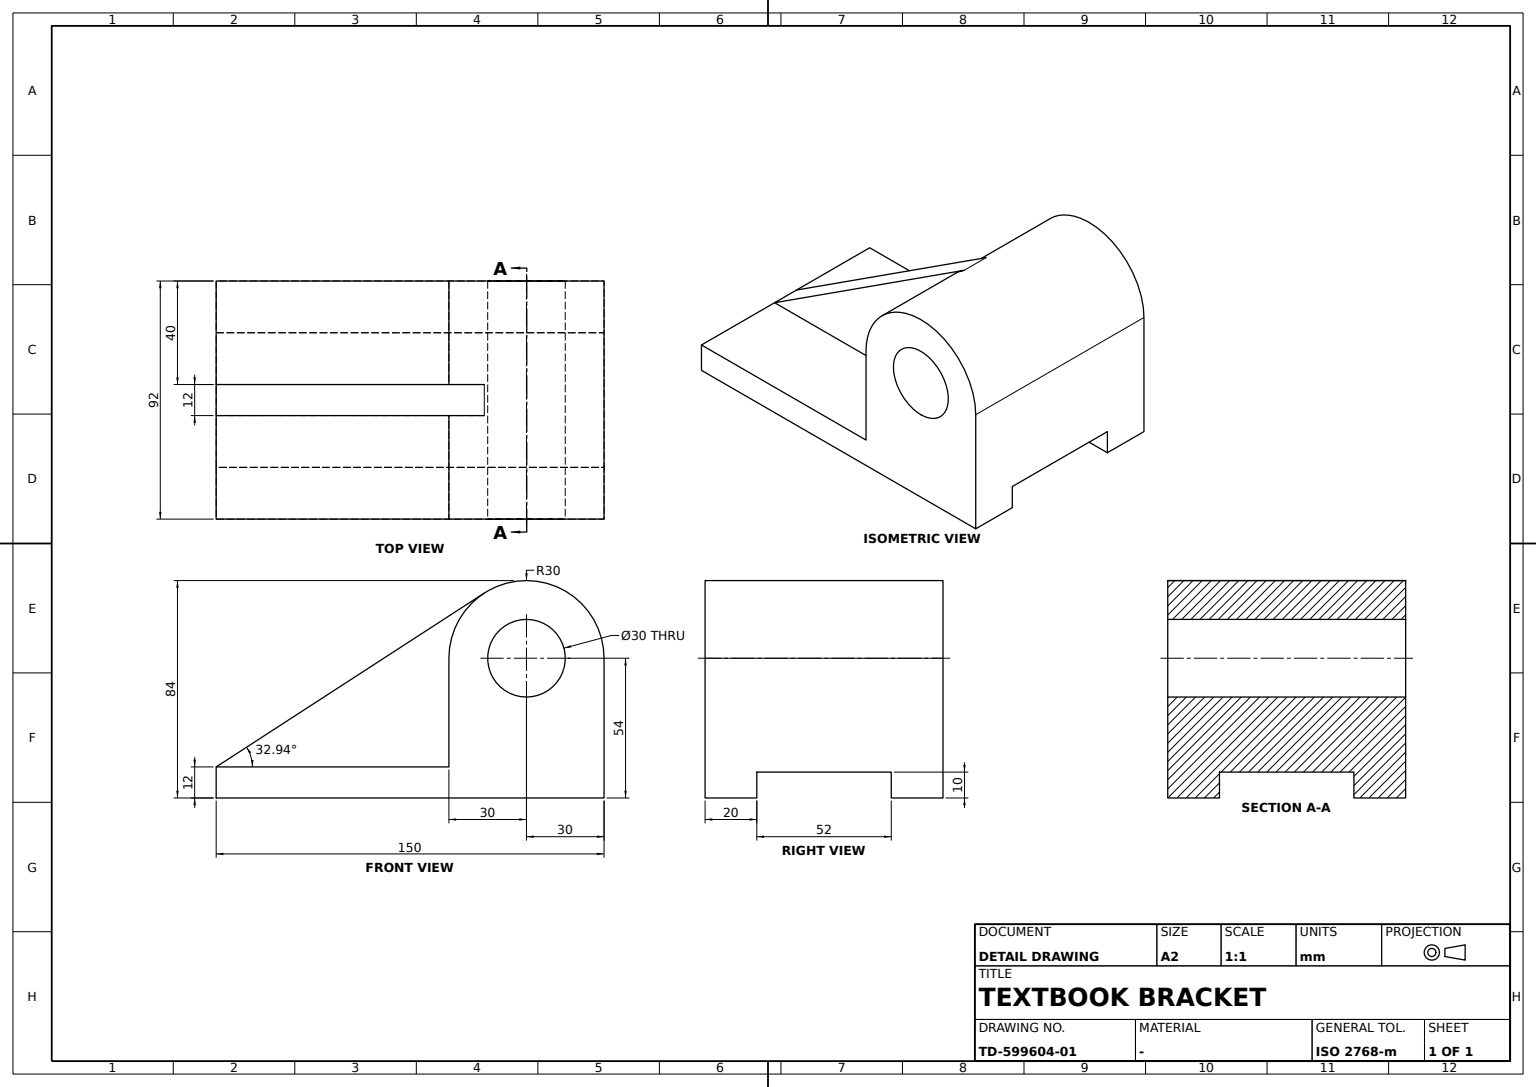
ISO-10303-21;
HEADER;
FILE_DESCRIPTION((''),'2;1');
FILE_NAME('','',(''),(''),'','','');
FILE_SCHEMA(('AUTOMOTIVE_DESIGN'));
ENDSEC;
DATA;
#1=APPLICATION_CONTEXT('');
#2=PRODUCT_CONTEXT('',#1,'mechanical');
#3=PRODUCT('','','',(#2));
#4=PRODUCT_DEFINITION_FORMATION('','',#3);
#5=PRODUCT_DEFINITION_CONTEXT('',#1,'design');
#6=PRODUCT_DEFINITION('','',#4,#5);
#7=PRODUCT_DEFINITION_SHAPE('','',#6);
#8=(LENGTH_UNIT()NAMED_UNIT(*)SI_UNIT(.MILLI.,.METRE.));
#9=(NAMED_UNIT(*)PLANE_ANGLE_UNIT()SI_UNIT($,.RADIAN.));
#10=(NAMED_UNIT(*)SI_UNIT($,.STERADIAN.)SOLID_ANGLE_UNIT());
#11=UNCERTAINTY_MEASURE_WITH_UNIT(LENGTH_MEASURE(0.005),#8,'distance_accuracy_value','');
#12=(GEOMETRIC_REPRESENTATION_CONTEXT(3)GLOBAL_UNCERTAINTY_ASSIGNED_CONTEXT((#11))GLOBAL_UNIT_ASSIGNED_CONTEXT((#8,#9,#10))REPRESENTATION_CONTEXT('',''));
#13=CARTESIAN_POINT('',(-26.,150.,10.));
#14=VERTEX_POINT('',#13);
#15=CARTESIAN_POINT('',(-26.,150.,0.));
#16=VERTEX_POINT('',#15);
#17=DIRECTION('',(0.,0.,-1.));
#18=VECTOR('',#17,1000.);
#19=LINE('',#13,#18);
#20=EDGE_CURVE('',#14,#16,#19,.T.);
#21=ORIENTED_EDGE('',*,*,#20,.F.);
#22=CARTESIAN_POINT('',(-26.,0.,10.));
#23=VERTEX_POINT('',#22);
#24=DIRECTION('',(0.,-1.,0.));
#25=VECTOR('',#24,1000.);
#26=LINE('',#13,#25);
#27=EDGE_CURVE('',#14,#23,#26,.T.);
#28=ORIENTED_EDGE('',*,*,#27,.T.);
#29=CARTESIAN_POINT('',(-26.,0.,0.));
#30=VERTEX_POINT('',#29);
#31=DIRECTION('',(0.,0.,1.));
#32=VECTOR('',#31,1000.);
#33=LINE('',#22,#32);
#34=EDGE_CURVE('',#30,#23,#33,.T.);
#35=ORIENTED_EDGE('',*,*,#34,.F.);
#36=LINE('',#15,#25);
#37=EDGE_CURVE('',#16,#30,#36,.T.);
#38=ORIENTED_EDGE('',*,*,#37,.F.);
#39=EDGE_LOOP('',(#21,#28,#35,#38));
#40=FACE_BOUND('',#39,.T.);
#41=DIRECTION('',(-1.,0.,0.));
#42=AXIS2_PLACEMENT_3D('',#13,#41,#17);
#43=PLANE('',#42);
#44=ADVANCED_FACE('',(#40),#43,.F.);
#45=CARTESIAN_POINT('',(6.,103.687829,79.177631));
#46=VERTEX_POINT('',#45);
#47=CARTESIAN_POINT('',(6.,90.,54.));
#48=VERTEX_POINT('',#47);
#49=CARTESIAN_POINT('',(6.,120.,54.));
#50=DIRECTION('',(1.,0.,0.));
#51=AXIS2_PLACEMENT_3D('',#49,#50,#17);
#52=CIRCLE('',#51,30.);
#53=EDGE_CURVE('',#46,#48,#52,.T.);
#54=ORIENTED_EDGE('',*,*,#53,.T.);
#55=CARTESIAN_POINT('',(46.,90.,54.));
#56=VERTEX_POINT('',#55);
#57=CARTESIAN_POINT('',(0.,90.,54.));
#58=VECTOR('',#50,1000.);
#59=LINE('',#57,#58);
#60=EDGE_CURVE('',#48,#56,#59,.T.);
#61=ORIENTED_EDGE('',*,*,#60,.T.);
#62=CARTESIAN_POINT('',(46.,150.,54.));
#63=VERTEX_POINT('',#62);
#64=CARTESIAN_POINT('',(46.,120.,54.));
#65=AXIS2_PLACEMENT_3D('',#64,#50,#17);
#66=CIRCLE('',#65,30.);
#67=EDGE_CURVE('',#63,#56,#66,.T.);
#68=ORIENTED_EDGE('',*,*,#67,.F.);
#69=CARTESIAN_POINT('',(-46.,150.,54.));
#70=VERTEX_POINT('',#69);
#71=CARTESIAN_POINT('',(0.,150.,54.));
#72=LINE('',#71,#58);
#73=EDGE_CURVE('',#70,#63,#72,.T.);
#74=ORIENTED_EDGE('',*,*,#73,.F.);
#75=CARTESIAN_POINT('',(-46.,90.,54.));
#76=VERTEX_POINT('',#75);
#77=CARTESIAN_POINT('',(-46.,120.,54.));
#78=AXIS2_PLACEMENT_3D('',#77,#50,#17);
#79=CIRCLE('',#78,30.);
#80=EDGE_CURVE('',#70,#76,#79,.T.);
#81=ORIENTED_EDGE('',*,*,#80,.T.);
#82=CARTESIAN_POINT('',(-6.,90.,54.));
#83=VERTEX_POINT('',#82);
#84=EDGE_CURVE('',#76,#83,#59,.T.);
#85=ORIENTED_EDGE('',*,*,#84,.T.);
#86=CARTESIAN_POINT('',(-6.,103.687829,79.177631));
#87=VERTEX_POINT('',#86);
#88=CARTESIAN_POINT('',(-6.,120.,54.));
#89=AXIS2_PLACEMENT_3D('',#88,#50,#17);
#90=CIRCLE('',#89,30.);
#91=EDGE_CURVE('',#87,#83,#90,.T.);
#92=ORIENTED_EDGE('',*,*,#91,.F.);
#93=CARTESIAN_POINT('',(0.,103.687829,79.177631));
#94=LINE('',#93,#58);
#95=EDGE_CURVE('',#87,#46,#94,.T.);
#96=ORIENTED_EDGE('',*,*,#95,.T.);
#97=EDGE_LOOP('',(#54,#61,#68,#74,#81,#85,#92,#96));
#98=FACE_BOUND('',#97,.T.);
#99=CARTESIAN_POINT('',(0.,120.,54.));
#100=DIRECTION('',(0.,1.,0.));
#101=AXIS2_PLACEMENT_3D('',#99,#50,#100);
#102=CYLINDRICAL_SURFACE('',#101,30.);
#103=ADVANCED_FACE('',(#98),#102,.T.);
#104=CARTESIAN_POINT('',(6.,90.,12.));
#105=VERTEX_POINT('',#104);
#106=CARTESIAN_POINT('',(6.,0.,12.));
#107=VERTEX_POINT('',#106);
#108=LINE('',#106,#25);
#109=EDGE_CURVE('',#105,#107,#108,.T.);
#110=ORIENTED_EDGE('',*,*,#109,.F.);
#111=CARTESIAN_POINT('',(6.,90.,0.));
#112=LINE('',#111,#18);
#113=EDGE_CURVE('',#48,#105,#112,.T.);
#114=ORIENTED_EDGE('',*,*,#113,.F.);
#115=ORIENTED_EDGE('',*,*,#53,.F.);
#116=DIRECTION('',(0.,-0.839254356,-0.543739024));
#117=VECTOR('',#116,1000.);
#118=LINE('',#45,#117);
#119=EDGE_CURVE('',#46,#107,#118,.T.);
#120=ORIENTED_EDGE('',*,*,#119,.T.);
#121=EDGE_LOOP('',(#110,#114,#115,#120));
#122=FACE_BOUND('',#121,.T.);
#123=CARTESIAN_POINT('',(6.,0.,0.));
#124=AXIS2_PLACEMENT_3D('',#123,#50,#100);
#125=PLANE('',#124);
#126=ADVANCED_FACE('',(#122),#125,.T.);
#127=CARTESIAN_POINT('',(-46.,0.,0.));
#128=VERTEX_POINT('',#127);
#129=CARTESIAN_POINT('',(-46.,150.,0.));
#130=VERTEX_POINT('',#129);
#131=VECTOR('',#100,1000.);
#132=LINE('',#127,#131);
#133=EDGE_CURVE('',#128,#130,#132,.T.);
#134=ORIENTED_EDGE('',*,*,#133,.T.);
#135=CARTESIAN_POINT('',(0.,150.,0.));
#136=LINE('',#135,#58);
#137=EDGE_CURVE('',#130,#16,#136,.T.);
#138=ORIENTED_EDGE('',*,*,#137,.T.);
#139=ORIENTED_EDGE('',*,*,#37,.T.);
#140=CARTESIAN_POINT('',(0.,0.,0.));
#141=LINE('',#140,#58);
#142=EDGE_CURVE('',#128,#30,#141,.T.);
#143=ORIENTED_EDGE('',*,*,#142,.F.);
#144=EDGE_LOOP('',(#134,#138,#139,#143));
#145=FACE_BOUND('',#144,.T.);
#146=AXIS2_PLACEMENT_3D('',#140,#17,#100);
#147=PLANE('',#146);
#148=ADVANCED_FACE('',(#145),#147,.T.);
#149=CARTESIAN_POINT('',(26.,150.,0.));
#150=VERTEX_POINT('',#149);
#151=CARTESIAN_POINT('',(26.,150.,10.));
#152=VERTEX_POINT('',#151);
#153=LINE('',#149,#32);
#154=EDGE_CURVE('',#150,#152,#153,.T.);
#155=ORIENTED_EDGE('',*,*,#154,.F.);
#156=CARTESIAN_POINT('',(26.,0.,0.));
#157=VERTEX_POINT('',#156);
#158=LINE('',#156,#25);
#159=EDGE_CURVE('',#150,#157,#158,.T.);
#160=ORIENTED_EDGE('',*,*,#159,.T.);
#161=CARTESIAN_POINT('',(26.,0.,10.));
#162=VERTEX_POINT('',#161);
#163=CARTESIAN_POINT('',(26.,0.,12.));
#164=LINE('',#163,#32);
#165=EDGE_CURVE('',#157,#162,#164,.T.);
#166=ORIENTED_EDGE('',*,*,#165,.T.);
#167=LINE('',#151,#25);
#168=EDGE_CURVE('',#152,#162,#167,.T.);
#169=ORIENTED_EDGE('',*,*,#168,.F.);
#170=EDGE_LOOP('',(#155,#160,#166,#169));
#171=FACE_BOUND('',#170,.T.);
#172=AXIS2_PLACEMENT_3D('',#149,#50,#31);
#173=PLANE('',#172);
#174=ADVANCED_FACE('',(#171),#173,.F.);
#175=CARTESIAN_POINT('',(46.,90.,12.));
#176=VERTEX_POINT('',#175);
#177=CARTESIAN_POINT('',(0.,90.,12.));
#178=LINE('',#177,#58);
#179=EDGE_CURVE('',#105,#176,#178,.T.);
#180=ORIENTED_EDGE('',*,*,#179,.T.);
#181=CARTESIAN_POINT('',(46.,90.,0.));
#182=LINE('',#181,#18);
#183=EDGE_CURVE('',#56,#176,#182,.T.);
#184=ORIENTED_EDGE('',*,*,#183,.F.);
#185=ORIENTED_EDGE('',*,*,#60,.F.);
#186=ORIENTED_EDGE('',*,*,#113,.T.);
#187=EDGE_LOOP('',(#180,#184,#185,#186));
#188=FACE_BOUND('',#187,.T.);
#189=AXIS2_PLACEMENT_3D('',#57,#24,#17);
#190=PLANE('',#189);
#191=ADVANCED_FACE('',(#188),#190,.T.);
#192=ORIENTED_EDGE('',*,*,#91,.T.);
#193=CARTESIAN_POINT('',(-6.,90.,12.));
#194=VERTEX_POINT('',#193);
#195=CARTESIAN_POINT('',(-6.,90.,0.));
#196=LINE('',#195,#18);
#197=EDGE_CURVE('',#83,#194,#196,.T.);
#198=ORIENTED_EDGE('',*,*,#197,.T.);
#199=CARTESIAN_POINT('',(-6.,0.,12.));
#200=VERTEX_POINT('',#199);
#201=LINE('',#199,#25);
#202=EDGE_CURVE('',#194,#200,#201,.T.);
#203=ORIENTED_EDGE('',*,*,#202,.T.);
#204=LINE('',#86,#117);
#205=EDGE_CURVE('',#87,#200,#204,.T.);
#206=ORIENTED_EDGE('',*,*,#205,.F.);
#207=EDGE_LOOP('',(#192,#198,#203,#206));
#208=FACE_BOUND('',#207,.T.);
#209=CARTESIAN_POINT('',(-6.,0.,0.));
#210=AXIS2_PLACEMENT_3D('',#209,#50,#100);
#211=PLANE('',#210);
#212=ADVANCED_FACE('',(#208),#211,.F.);
#213=ORIENTED_EDGE('',*,*,#27,.F.);
#214=VECTOR('',#41,1000.);
#215=LINE('',#151,#214);
#216=EDGE_CURVE('',#152,#14,#215,.T.);
#217=ORIENTED_EDGE('',*,*,#216,.F.);
#218=ORIENTED_EDGE('',*,*,#168,.T.);
#219=CARTESIAN_POINT('',(0.,0.,10.));
#220=LINE('',#219,#214);
#221=EDGE_CURVE('',#162,#23,#220,.T.);
#222=ORIENTED_EDGE('',*,*,#221,.T.);
#223=EDGE_LOOP('',(#213,#217,#218,#222));
#224=FACE_BOUND('',#223,.T.);
#225=AXIS2_PLACEMENT_3D('',#151,#31,#41);
#226=PLANE('',#225);
#227=ADVANCED_FACE('',(#224),#226,.F.);
#228=ORIENTED_EDGE('',*,*,#109,.T.);
#229=CARTESIAN_POINT('',(46.,0.,12.));
#230=VERTEX_POINT('',#229);
#231=CARTESIAN_POINT('',(0.,0.,12.));
#232=LINE('',#231,#58);
#233=EDGE_CURVE('',#107,#230,#232,.T.);
#234=ORIENTED_EDGE('',*,*,#233,.T.);
#235=LINE('',#229,#25);
#236=EDGE_CURVE('',#176,#230,#235,.T.);
#237=ORIENTED_EDGE('',*,*,#236,.F.);
#238=ORIENTED_EDGE('',*,*,#179,.F.);
#239=EDGE_LOOP('',(#228,#234,#237,#238));
#240=FACE_BOUND('',#239,.T.);
#241=AXIS2_PLACEMENT_3D('',#177,#31,#24);
#242=PLANE('',#241);
#243=ADVANCED_FACE('',(#240),#242,.T.);
#244=CARTESIAN_POINT('',(-46.,0.,12.));
#245=VERTEX_POINT('',#244);
#246=LINE('',#127,#18);
#247=EDGE_CURVE('',#245,#128,#246,.T.);
#248=ORIENTED_EDGE('',*,*,#247,.F.);
#249=CARTESIAN_POINT('',(-46.,90.,12.));
#250=VERTEX_POINT('',#249);
#251=LINE('',#244,#25);
#252=EDGE_CURVE('',#250,#245,#251,.T.);
#253=ORIENTED_EDGE('',*,*,#252,.F.);
#254=CARTESIAN_POINT('',(-46.,90.,0.));
#255=LINE('',#254,#18);
#256=EDGE_CURVE('',#76,#250,#255,.T.);
#257=ORIENTED_EDGE('',*,*,#256,.F.);
#258=ORIENTED_EDGE('',*,*,#80,.F.);
#259=LINE('',#129,#32);
#260=EDGE_CURVE('',#130,#70,#259,.T.);
#261=ORIENTED_EDGE('',*,*,#260,.F.);
#262=ORIENTED_EDGE('',*,*,#133,.F.);
#263=EDGE_LOOP('',(#248,#253,#257,#258,#261,#262));
#264=FACE_BOUND('',#263,.T.);
#265=CARTESIAN_POINT('',(-46.,120.,39.));
#266=VERTEX_POINT('',#265);
#267=CIRCLE('',#78,15.);
#268=EDGE_CURVE('',#266,#266,#267,.T.);
#269=ORIENTED_EDGE('',*,*,#268,.T.);
#270=EDGE_LOOP('',(#269));
#271=FACE_BOUND('',#270,.T.);
#272=AXIS2_PLACEMENT_3D('',#127,#50,#100);
#273=PLANE('',#272);
#274=ADVANCED_FACE('',(#264,#271),#273,.F.);
#275=ORIENTED_EDGE('',*,*,#84,.F.);
#276=ORIENTED_EDGE('',*,*,#256,.T.);
#277=EDGE_CURVE('',#250,#194,#178,.T.);
#278=ORIENTED_EDGE('',*,*,#277,.T.);
#279=ORIENTED_EDGE('',*,*,#197,.F.);
#280=EDGE_LOOP('',(#275,#276,#278,#279));
#281=FACE_BOUND('',#280,.T.);
#282=ADVANCED_FACE('',(#281),#190,.T.);
#283=CARTESIAN_POINT('',(46.,120.,39.));
#284=VERTEX_POINT('',#283);
#285=CIRCLE('',#65,15.);
#286=EDGE_CURVE('',#284,#284,#285,.T.);
#287=ORIENTED_EDGE('',*,*,#286,.F.);
#288=EDGE_LOOP('',(#287));
#289=FACE_BOUND('',#288,.T.);
#290=CARTESIAN_POINT('',(46.,0.,0.));
#291=VERTEX_POINT('',#290);
#292=LINE('',#290,#18);
#293=EDGE_CURVE('',#230,#291,#292,.T.);
#294=ORIENTED_EDGE('',*,*,#293,.T.);
#295=CARTESIAN_POINT('',(46.,150.,0.));
#296=VERTEX_POINT('',#295);
#297=LINE('',#290,#131);
#298=EDGE_CURVE('',#291,#296,#297,.T.);
#299=ORIENTED_EDGE('',*,*,#298,.T.);
#300=LINE('',#295,#32);
#301=EDGE_CURVE('',#296,#63,#300,.T.);
#302=ORIENTED_EDGE('',*,*,#301,.T.);
#303=ORIENTED_EDGE('',*,*,#67,.T.);
#304=ORIENTED_EDGE('',*,*,#183,.T.);
#305=ORIENTED_EDGE('',*,*,#236,.T.);
#306=EDGE_LOOP('',(#294,#299,#302,#303,#304,#305));
#307=FACE_BOUND('',#306,.T.);
#308=AXIS2_PLACEMENT_3D('',#290,#50,#100);
#309=PLANE('',#308);
#310=ADVANCED_FACE('',(#289,#307),#309,.T.);
#311=EDGE_CURVE('',#157,#291,#141,.T.);
#312=ORIENTED_EDGE('',*,*,#311,.T.);
#313=ORIENTED_EDGE('',*,*,#293,.F.);
#314=ORIENTED_EDGE('',*,*,#233,.F.);
#315=EDGE_CURVE('',#200,#107,#232,.T.);
#316=ORIENTED_EDGE('',*,*,#315,.F.);
#317=EDGE_CURVE('',#245,#200,#232,.T.);
#318=ORIENTED_EDGE('',*,*,#317,.F.);
#319=ORIENTED_EDGE('',*,*,#247,.T.);
#320=ORIENTED_EDGE('',*,*,#142,.T.);
#321=ORIENTED_EDGE('',*,*,#34,.T.);
#322=ORIENTED_EDGE('',*,*,#221,.F.);
#323=ORIENTED_EDGE('',*,*,#165,.F.);
#324=EDGE_LOOP('',(#312,#313,#314,#316,#318,#319,#320,#321,#322,#323));
#325=FACE_BOUND('',#324,.T.);
#326=AXIS2_PLACEMENT_3D('',#231,#24,#17);
#327=PLANE('',#326);
#328=ADVANCED_FACE('',(#325),#327,.T.);
#329=ORIENTED_EDGE('',*,*,#159,.F.);
#330=EDGE_CURVE('',#150,#296,#136,.T.);
#331=ORIENTED_EDGE('',*,*,#330,.T.);
#332=ORIENTED_EDGE('',*,*,#298,.F.);
#333=ORIENTED_EDGE('',*,*,#311,.F.);
#334=EDGE_LOOP('',(#329,#331,#332,#333));
#335=FACE_BOUND('',#334,.T.);
#336=ADVANCED_FACE('',(#335),#147,.T.);
#337=ORIENTED_EDGE('',*,*,#315,.T.);
#338=ORIENTED_EDGE('',*,*,#119,.F.);
#339=ORIENTED_EDGE('',*,*,#95,.F.);
#340=ORIENTED_EDGE('',*,*,#205,.T.);
#341=EDGE_LOOP('',(#337,#338,#339,#340));
#342=FACE_BOUND('',#341,.T.);
#343=DIRECTION('',(0.,0.543739024,-0.839254356));
#344=DIRECTION('',(0.,0.839254356,0.543739024));
#345=AXIS2_PLACEMENT_3D('',#93,#343,#344);
#346=PLANE('',#345);
#347=ADVANCED_FACE('',(#342),#346,.F.);
#348=ORIENTED_EDGE('',*,*,#330,.F.);
#349=ORIENTED_EDGE('',*,*,#154,.T.);
#350=ORIENTED_EDGE('',*,*,#216,.T.);
#351=ORIENTED_EDGE('',*,*,#20,.T.);
#352=ORIENTED_EDGE('',*,*,#137,.F.);
#353=ORIENTED_EDGE('',*,*,#260,.T.);
#354=ORIENTED_EDGE('',*,*,#73,.T.);
#355=ORIENTED_EDGE('',*,*,#301,.F.);
#356=EDGE_LOOP('',(#348,#349,#350,#351,#352,#353,#354,#355));
#357=FACE_BOUND('',#356,.T.);
#358=AXIS2_PLACEMENT_3D('',#135,#100,#31);
#359=PLANE('',#358);
#360=ADVANCED_FACE('',(#357),#359,.T.);
#361=ORIENTED_EDGE('',*,*,#202,.F.);
#362=ORIENTED_EDGE('',*,*,#277,.F.);
#363=ORIENTED_EDGE('',*,*,#252,.T.);
#364=ORIENTED_EDGE('',*,*,#317,.T.);
#365=EDGE_LOOP('',(#361,#362,#363,#364));
#366=FACE_BOUND('',#365,.T.);
#367=ADVANCED_FACE('',(#366),#242,.T.);
#368=ORIENTED_EDGE('',*,*,#286,.T.);
#369=EDGE_LOOP('',(#368));
#370=FACE_BOUND('',#369,.T.);
#371=ORIENTED_EDGE('',*,*,#268,.F.);
#372=EDGE_LOOP('',(#371));
#373=FACE_BOUND('',#372,.T.);
#374=CYLINDRICAL_SURFACE('',#101,15.);
#375=ADVANCED_FACE('',(#370,#373),#374,.F.);
#376=CLOSED_SHELL('',(#44,#103,#126,#148,#174,#191,#212,#227,#243,#274,#282,#310,#328,#336,#347,#360,#367,#375));
#377=MANIFOLD_SOLID_BREP('',#376);
#378=ADVANCED_BREP_SHAPE_REPRESENTATION('',(#377),#12);
#379=SHAPE_DEFINITION_REPRESENTATION(#7,#378);
ENDSEC;
END-ISO-10303-21;
